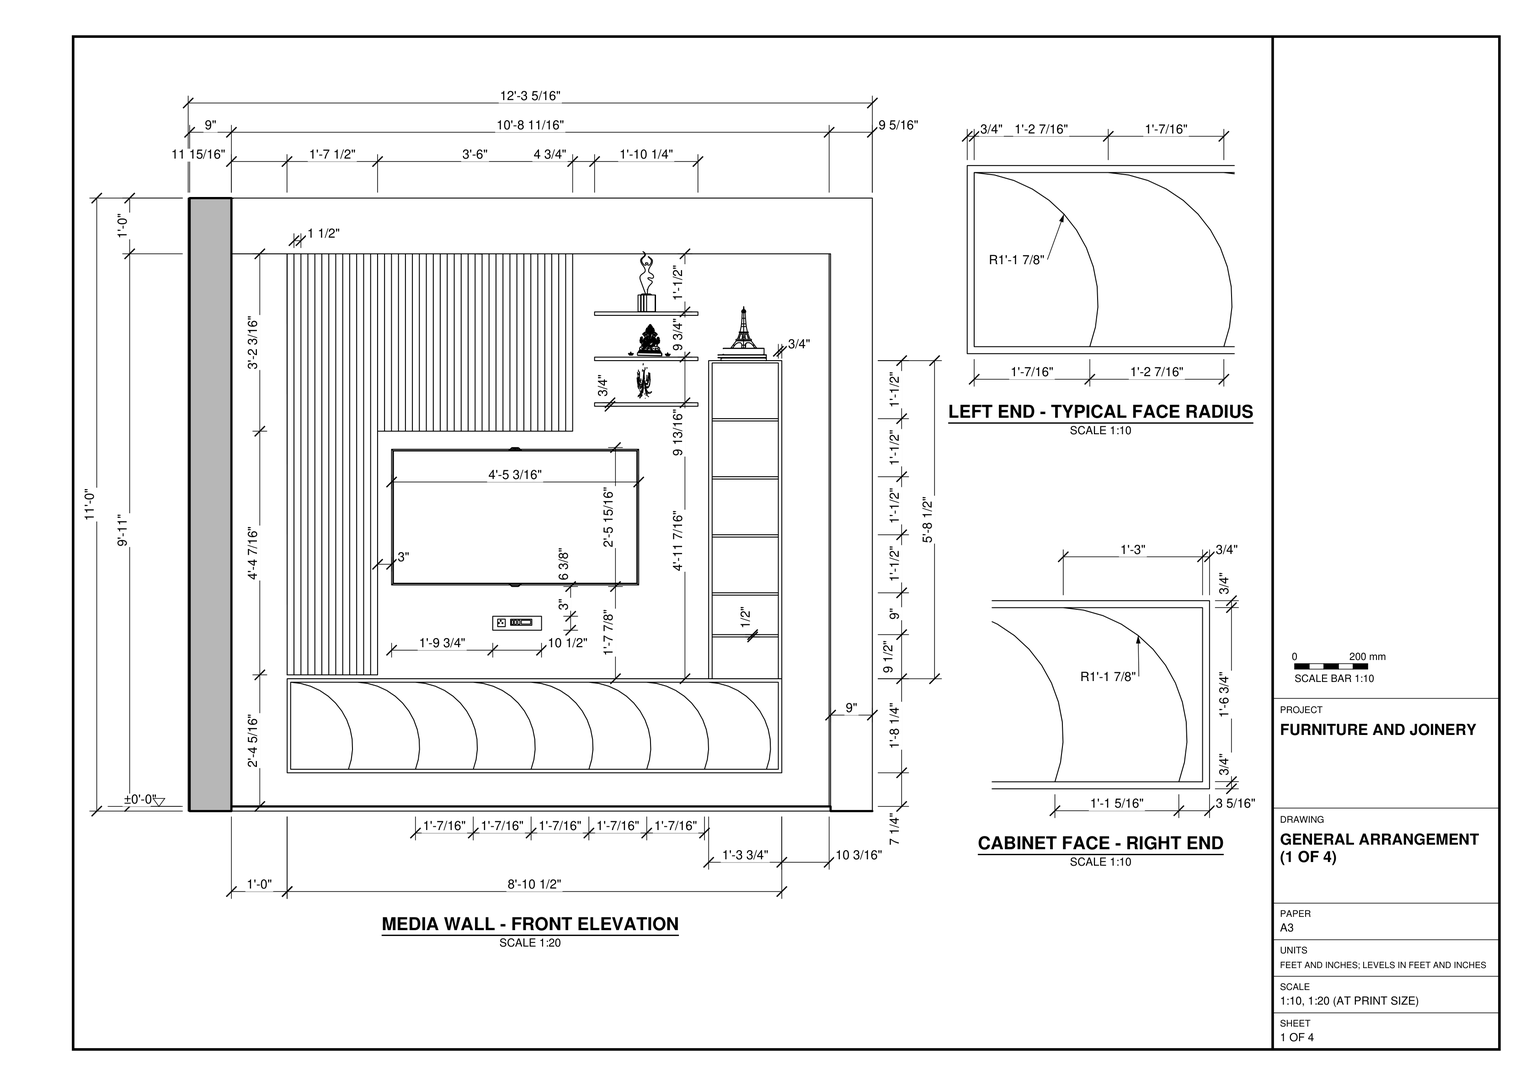
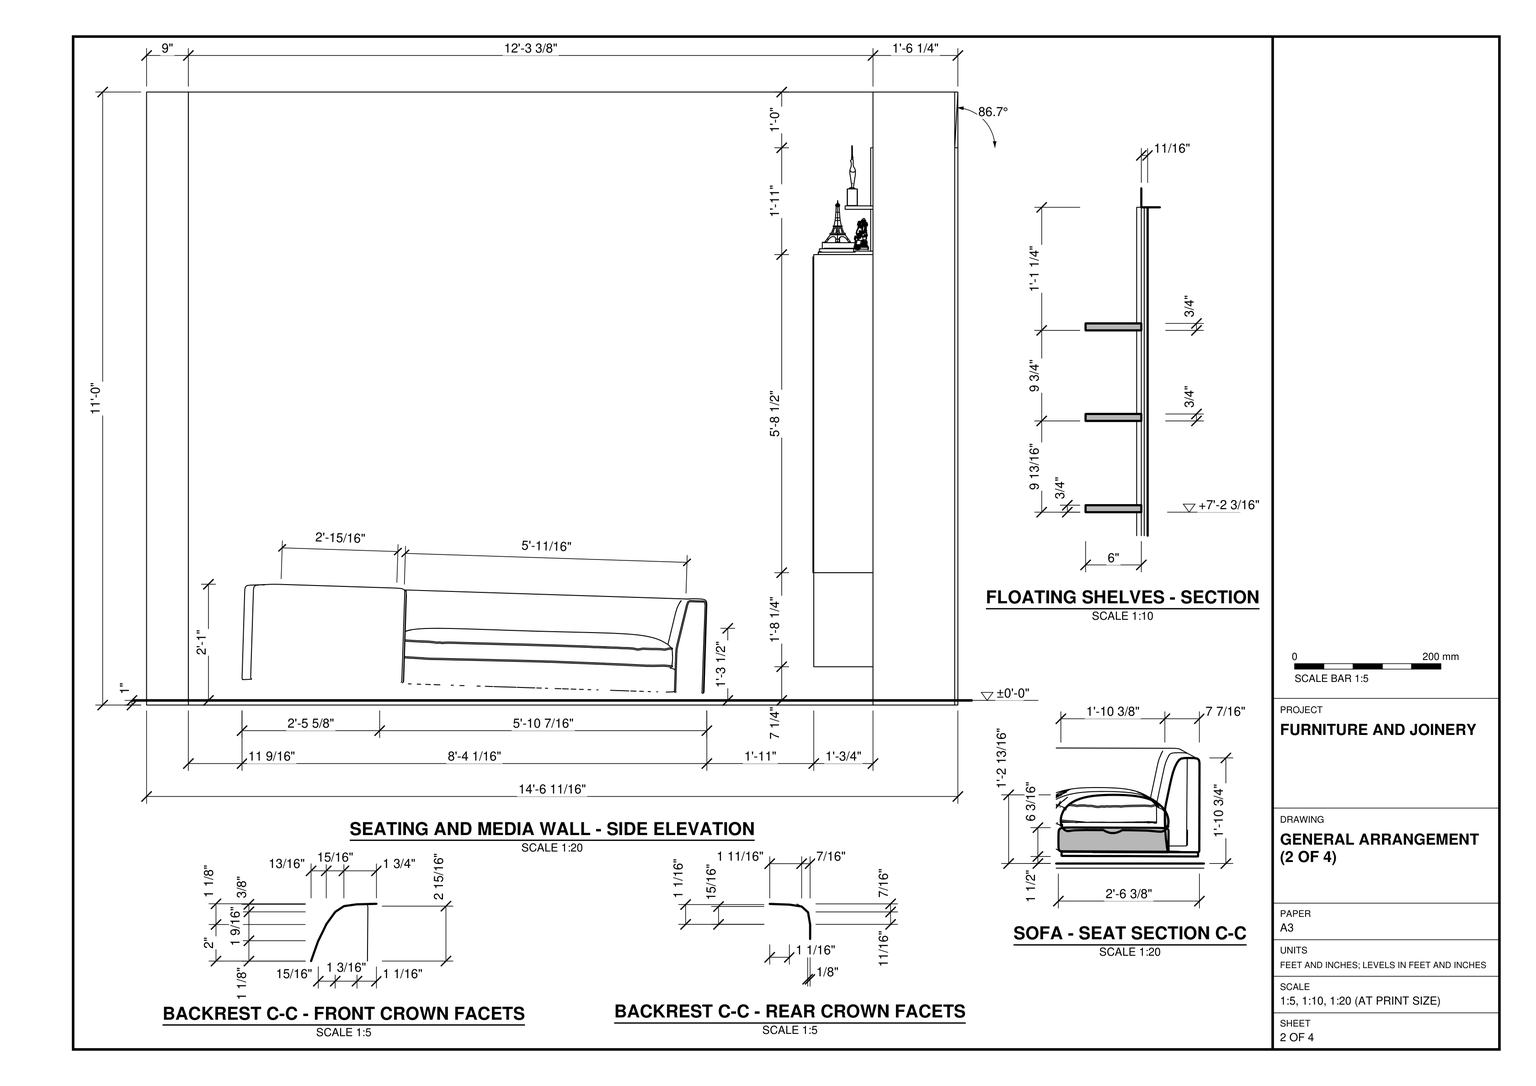
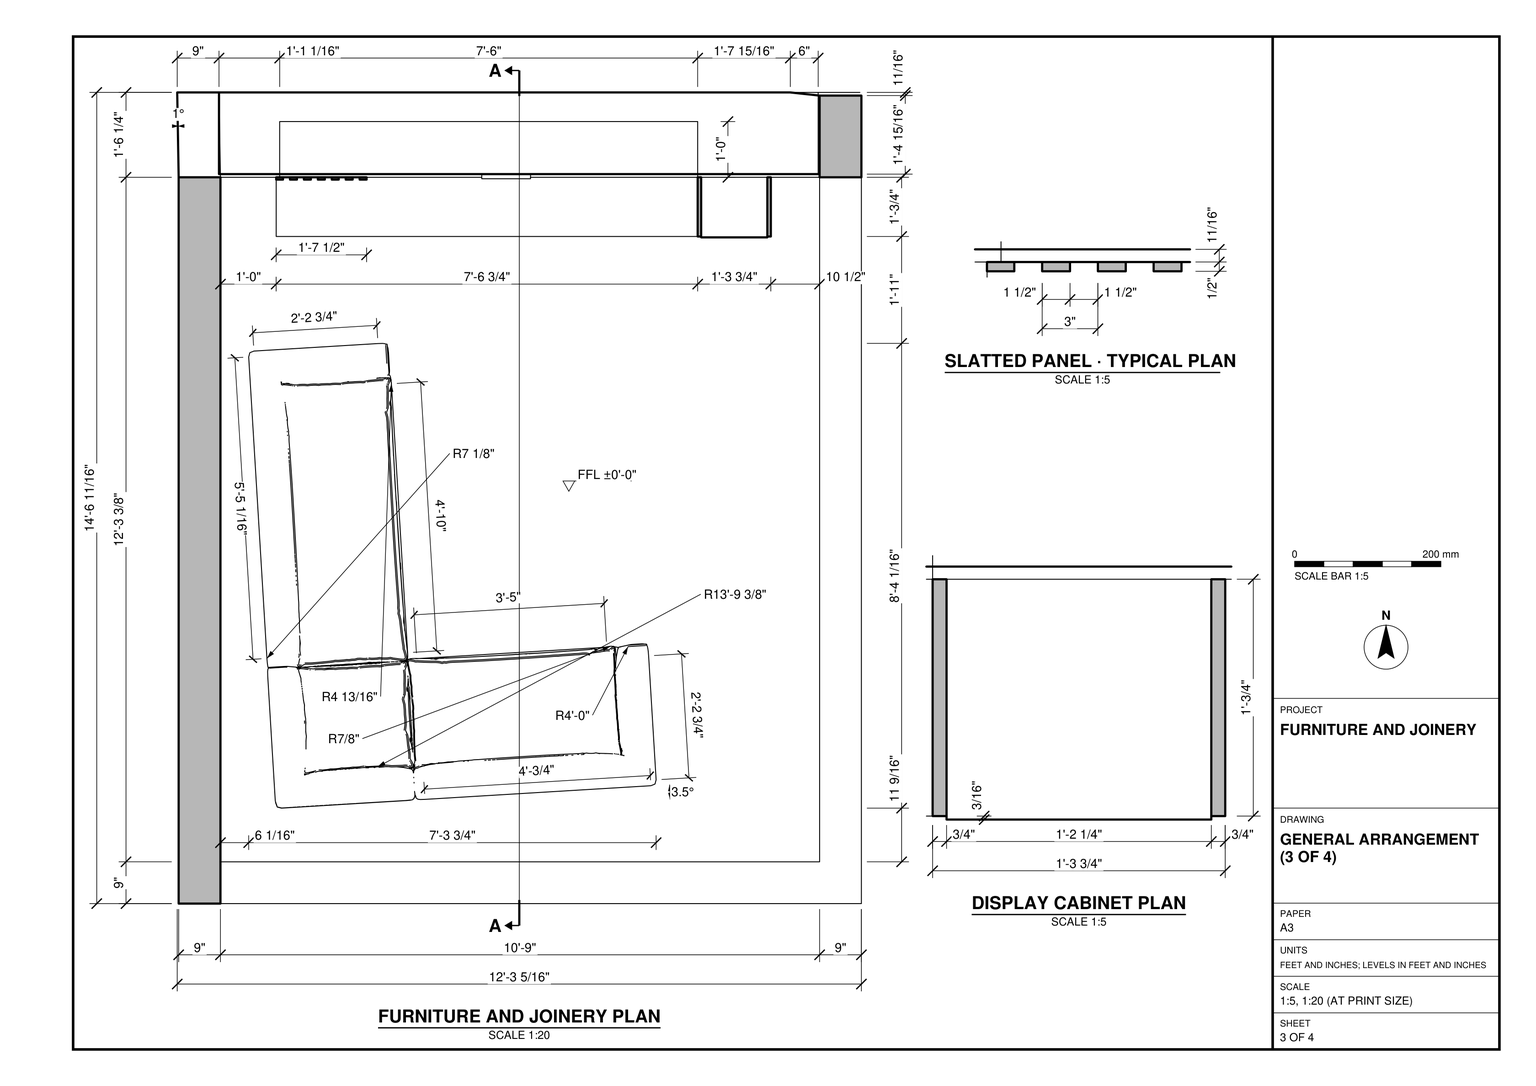
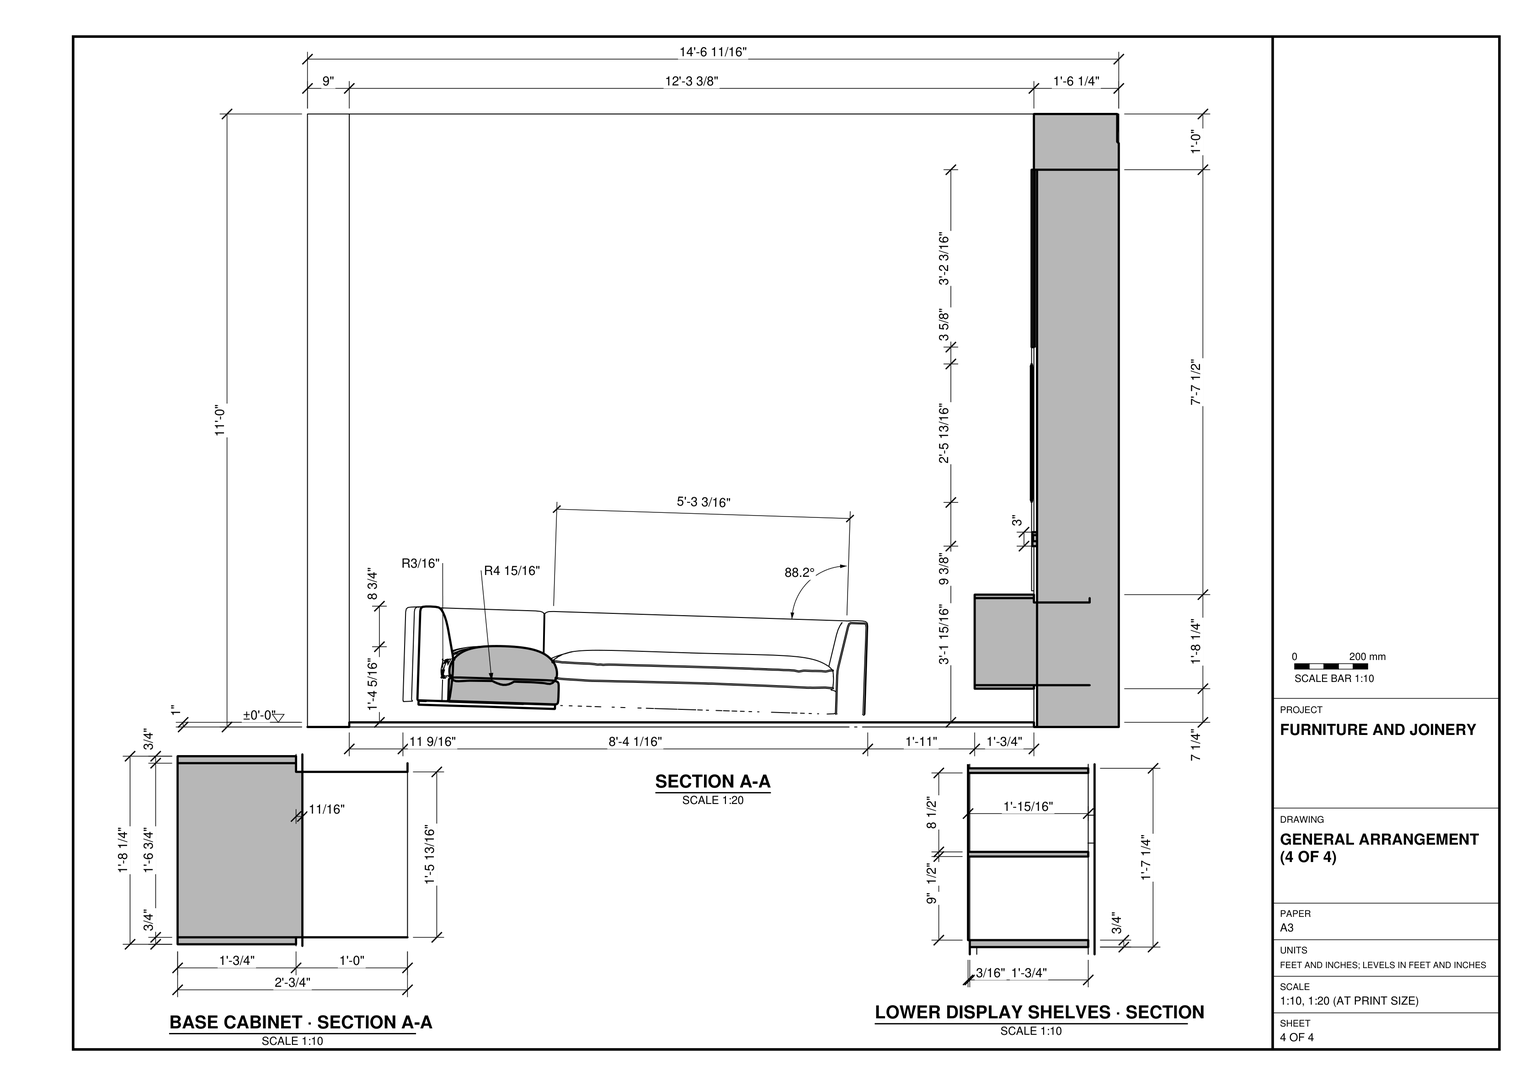
Build the seating area in SketchUp using task_files/diagram_01.pdf. Work in feet and inches. The overall model is 12'-3 5/16" wide by 14'-6 11/16" deep by 11'-2" high, with the finished floor at ±0'-0". Model the floor, the 9" left wall and the media-wall surround, following the plan and sections for their thicknesses and returns.

Set the long base cabinet above the floor and form its fronts with the repeated curved edges shown in the end details. Above it, run the vertical slats down the left side of the screen and across the area above it, keeping the stepped lower edge shown in elevation. Place the outlet plate below the screen. Fit the open display cabinet at the right end of the base cabinet and the three floating shelves between the slatted panel and the display cabinet.

Build the L-shaped sectional sofa with the seat and back profiles shown in section. Position its long leg near the left wall and its shorter leg across the room, preserving the slight angle shown in plan. Decor and loose items may be any suitable library components. Keep shell elements and individual furniture and joinery pieces in separate groups or components, and use components for repeated parts. Save one SketchUp model as output_files/seating_area_with_a_fitted_media_wall.skp.

# SketchUp Ruby script. Lengths in inches.
U = 1.inch
M = Sketchup.active_model
def pt(a) = Geom::Point3d.new(a.map { |v| v * U })
def face(e, loops, mat)
  f = e.add_face(loops[0].map { |a| pt(a) })
  loops[1..].each { |l| e.add_face(l.map { |a| pt(a) }).erase! }
  f.material = f.back_material = mat if mat
  f
end
# faces: each face lists its corners as indices into pts; further lists are holes
def faces(e, pts, list, mat = nil) = list.each { |f| face(e, (f[0].is_a?(Array) ? f : [f]).map { |l| l.map { |i| pts[i] } }, mat) }
# xy, xz, yz: faces in a plane at the given z, y or x. An outline is a flat list of corners, or four numbers for a rectangle; further outlines are holes
def ring(l) = l.size == 4 ? [[l[0], l[1]], [l[2], l[1]], [l[2], l[3]], [l[0], l[3]]] : l.each_slice(2).to_a
def flat(e, list, mat, &to3) = list.each { |f| face(e, (f[0].is_a?(Array) ? f : [f]).map { |l| ring(l).map { |u, v| to3.(u, v) } }, mat) }
def xy(e, z, list, mat = nil) = flat(e, list, mat) { |x, y| [x, y, z] }
def xz(e, y, list, mat = nil) = flat(e, list, mat) { |x, z| [x, y, z] }
def yz(e, x, list, mat = nil) = flat(e, list, mat) { |y, z| [x, y, z] }
def lines(e, pts, list) = list.each { |a, b| e.add_line(pt(pts[a]), pt(pts[b])) }
# prism: a flat outline (further loops are holes) pulled along v
def prism(e, loops, v, mat = nil)
  f = face(e, loops, mat); d = Geom::Vector3d.new(v.map { |x| x * U })
  f.pushpull(f.normal.samedirection?(d) ? d.length : -d.length)
end
def box(e, o, s, mat = nil) = prism(e, [[o, [o[0] + s[0], o[1], o[2]], [o[0] + s[0], o[1] + s[1], o[2]], [o[0], o[1] + s[1], o[2]]]], [0, 0, s[2]], mat)
def at(x, y, z, deg = 0) = Geom::Transformation.translation(pt([x, y, z])) * Geom::Transformation.rotation(ORIGIN, Z_AXIS, deg.degrees)
def axes(o, x, y, z) = Geom::Transformation.new([*x, 0, *y, 0, *z, 0, *pt(o).to_a, 1])
def part(name) = M.definitions.add(name)
# library, detail: a bought-in or finely detailed component or shape, given as its bounding box
def library(name, o, s) = part(name).tap { |d| box(d.entities, o, s) }
def detail(e, o, s) = box(e.add_group.entities, o, s)
def put(e, d, t, mat = nil) = e.add_instance(d, t).tap { |i| i.material = mat if mat }
def group(e, t, mat = nil) = e.add_group.tap { |g| g.transformation = t; g.material = mat if mat }.entities
root = M.entities
M.materials.add("01 - Default2").color = [86, 82, 73]
M.materials.add("6159 FRENCH NUT TREE").color = [139, 95, 49]
M.materials.add("6165 white ash").color = [208, 202, 179]
M.materials.add("6168 WARM ASH").color = [112, 88, 70]
M.materials.add("6184 Aged Elm").color = [88, 77, 65]
M.materials.add("6208 Grey Limed Oak1").color = [150, 141, 131]
M.materials.add("6220 Light Classic Oak").color = [174, 147, 110]
M.materials.add("Heather_Brim1").color = [51, 32, 20]
M.materials.add("Heather_Jeans").color = [86, 117, 147]
M.materials.add("Heather_PantShadow").color = [42, 79, 119]
M.materials.add("Heather_Skin").color = [221, 149, 116]
M.materials.add("Lily_Blonde").color = [204, 166, 108]
M.materials["Lily_Blonde"].alpha = 0.96
M.materials.add("Lily_Light").color = [226, 229, 211]
M.materials.add("Material \#21474428082").color = [180, 179, 173]
M.materials.add("Material \#3a2").color = [91, 47, 14]
M.materials.add("Material~1").color = [48, 234, 223]
M.materials["Material~1"].alpha = 0.35
M.materials.add("[Water Sparkling]").color = [216, 155, 0]
M.materials["[Water Sparkling]"].alpha = 0.6
c1 = library("Flat screen television",[-0.12,1.28,1.14],[53.2,0.41,29.93])
c2 = library("Books with figurine",[-0.1,-1.02,0],[11.3,11.3,11.77])
c3 = library("05 deco",[0,0,0],[11.39,11.6,68.34])
c4 = library("Statue with lamps",[-8.78,0,0],[8.78,25.04,18.65])
c5 = library("Assembly~89_Defintion\#1",[-458.17,-402.78,-169.48],[856.22,828.13,1000])
c6 = library("sofa+(2)",[-221.02,245.34,-31.11],[88.4,103.18,30.14])
xy(root,0,[[0.313,0,9.313,156.404],[0.313,156.404,9.313,156.404,9,174.681,0,174.681],[9.313,156.404,9,174.681,132,174.681,138.313,174,138.313,156.404],[138.313,156.404,147.313,174]],"Lily_Light")
xy(root,0,[[9.313,0,147.313,0,147.313,156.404,138.313,156.404,138.313,9,9.313,9]],"Material \#21474428082")
xy(root,1,[[9.313,9,138.313,156.404]],"Material \#21474428082")
xy(root,8.25,[[21.313,143.654,112.813,156.404],[112.813,143.654,127.813,156.404]])
xy(root,9,[[22.063,143.654,112.063,143.654,112.063,156.404,21.313,156.404,21.313,144.404,22.063,144.404],[112.813,143.654,127.063,156.404],[22.063,156.404,112.063,168.404]])
xy(root,26.8125,[[22.063,156.404,112.063,168.404]])
xy(root,27.75,[[22.063,143.654,22.063,144.404,21.313,144.404,21.313,156.404,112.063,156.404,112.063,143.654],[112.813,143.654,127.063,156.404]])
xy(root,28.5,[[112.813,143.467,127.063,143.654],[112.063,143.654,112.813,156.404],[112.813,143.654,127.063,156.404],[127.063,143.654,127.813,156.404]])
xy(root,28.5,[[21.313,143.654,112.063,156.404]],"6165 white ash")
xy(root,29.338,[[21.313,155.904,22.778,156.404],[24.278,155.904,25.778,156.404],[27.278,155.904,28.778,156.404]],"Heather_Brim1")
xy(root,29.338,[[30.278,155.904,31.778,156.404],[33.278,155.904,34.778,156.404],[36.278,155.904,37.778,156.404],[39.278,155.904,40.778,156.404]],"Lily_Light")
xy(root,37.5,[[112.813,143.467,127.063,156.404]])
xy(root,38,[[112.813,143.467,127.063,156.404]])
xy(root,38.949,[[65.577,156.086,76.077,157.086]])
xy(root,39.71,[[66.641,156.086,68.266,156.273],[66.641,156.273,68.266,157.086]])
xy(root,40.003,[[69.426,156.086,73.989,156.211],[69.426,156.211,73.989,157.086]])
xy(root,41.315,[[69.426,156.086,73.989,156.211],[69.426,156.211,73.989,157.086]])
xy(root,41.335,[[66.641,156.086,68.266,156.273],[66.641,156.273,68.266,157.086]])
xy(root,41.949,[[65.577,156.086,76.077,157.086]])
xy(root,46.5,[[112.813,143.467,127.063,156.404]])
xy(root,47,[[112.813,143.467,127.063,156.404]])
xy(root,59,[[112.813,143.467,127.063,156.404]])
xy(root,59.5,[[112.813,143.467,127.063,156.404]])
xy(root,71.5,[[112.813,143.467,127.063,156.404]])
xy(root,72,[[112.813,143.467,127.063,156.404]])
xy(root,81.804,[[42.278,155.904,43.778,156.404],[45.278,155.904,46.778,156.404],[48.278,155.904,49.778,156.404],[51.278,155.904,52.778,156.404],[54.278,155.904,55.778,156.404],
  [57.278,155.904,58.778,156.404],[60.278,155.904,61.778,156.717],[63.278,155.904,64.778,156.404],[66.278,155.904,67.778,156.404],[69.278,155.904,70.778,156.404],
  [72.278,155.904,73.778,156.404],[75.278,155.904,76.778,156.404],[78.278,155.904,79.778,156.404],[81.278,155.904,82.778,156.404]],"Lily_Light")
xy(root,84,[[112.813,143.467,127.063,156.404]])
xy(root,84.5,[[112.813,143.467,127.063,156.404]])
xy(root,87.175,[[87.5,150.404,109.757,156.404]],"Heather_PantShadow")
xy(root,87.925,[[87.5,150.404,109.757,156.404]],"6208 Grey Limed Oak1")
xy(root,96.5,[[112.813,143.467,127.063,143.654],[112.813,143.654,127.063,156.404]])
xy(root,97,[[112.063,143.654,127.813,156.404]],"6165 white ash")
xy(root,97,[[87.5,150.404,109.757,156.404]],"Heather_PantShadow")
xy(root,97.75,[[87.5,150.404,109.757,156.404]],"6208 Grey Limed Oak1")
xy(root,106.75,[[87.5,150.404,109.757,156.404]],"Heather_PantShadow")
xy(root,107.5,[[87.5,150.404,109.757,156.404]],"6208 Grey Limed Oak1")
xy(root,120,[[21.278,155.904,22.778,156.404],[24.278,155.904,25.778,156.404],[27.278,155.904,28.778,156.404]],"Heather_Brim1")
xy(root,120,[[30.278,155.904,31.778,156.404],[33.278,155.904,34.778,156.404],[36.278,155.904,37.778,156.404],[39.278,155.904,40.778,156.404],[42.278,155.904,43.778,156.404],
  [45.278,155.904,46.778,156.404],[48.278,155.904,49.778,156.404],[51.278,155.904,52.778,156.404],[54.278,155.904,55.778,156.404],[57.278,155.904,58.778,156.404],
  [60.278,155.904,61.778,156.404],[63.278,155.904,64.778,156.404],[66.278,155.904,67.778,156.404],[69.278,155.904,70.778,156.404],[72.278,155.904,73.778,156.404],
  [75.278,155.904,76.778,156.404],[78.278,155.904,79.778,156.404],[81.278,155.904,82.778,156.404],[9.313,156.404,60.278,156.404,60.278,156.717,61.778,156.717,61.778,156.404,138.313,156.404,138.313,174,132,174.681,9,174.681],[60.278,156.404,61.778,156.717]],"Lily_Light")
xy(root,132,[[0.313,0,9.313,156.404],[0.313,156.404,9.313,156.404,9,174.681,0,174.681],[9.313,156.404,147.313,156.404,147.313,174,138.313,174,9,174.681]],"Lily_Light")
xz(root,0,[[0.313,0,9.313,132]],"Lily_Light")
xz(root,9,[[9.313,0,138.313,1]],"Lily_Light")
xz(root,143.467,[[112.813,37.5,127.063,38],[112.813,46.5,127.063,47],[112.813,59,127.063,59.5],[112.813,71.5,127.063,72],[112.813,84,127.063,84.5]],"Lily_Blonde")
xz(root,143.467,[[112.813,28.5,127.063,37.5],[112.813,38,127.063,46.5],[112.813,47,127.063,59],[112.813,59.5,127.063,71.5],[112.813,72,127.063,84],
  [112.813,84.5,127.063,96.5]],"Material~1")
xz(root,143.654,[[124.509,9,127.063,9,127.063,27.75,112.063,27.75,114.232,27.491,116.334,26.896,118.316,25.978,120.129,24.761,121.73,23.274,123.077,21.555,124.138,19.646,124.887,17.594,125.304,15.45,125.38,13.267,125.113,11.099]],"01 - Default2")
xz(root,143.654,[[22.063,9,34.509,9,35.113,11.099,35.38,13.267,35.304,15.45,34.887,17.594,34.138,19.646,33.077,21.555,31.73,23.274,30.129,24.761,28.316,25.978,26.334,26.896,24.232,27.491,22.063,27.75],[34.509,9,48.939,9,49.543,11.099,49.81,13.267,49.734,15.45,49.316,17.594,48.568,19.646,47.507,21.555,46.159,23.274,44.559,24.761,42.745,25.978,40.763,26.896,38.662,27.491,36.493,27.75,22.063,27.75,24.232,27.491,26.334,26.896,28.316,25.978,30.129,24.761,31.73,23.274,33.077,21.555,34.138,19.646,34.887,17.594,35.304,15.45,35.38,13.267,35.113,11.099],[48.939,9,61.385,9,61.989,11.099,62.256,13.267,62.18,15.45,61.762,17.594,61.014,19.646,59.953,21.555,58.605,23.274,57.005,24.761,55.191,25.978,53.209,26.896,51.108,27.491,48.939,27.75,36.493,27.75,38.662,27.491,40.763,26.896,42.745,25.978,44.559,24.761,46.159,23.274,47.507,21.555,48.568,19.646,49.316,17.594,49.734,15.45,49.81,13.267,49.543,11.099],[61.385,9,73.831,9,74.435,11.099,74.702,13.267,74.626,15.45,74.208,17.594,73.46,19.646,72.399,21.555,71.051,23.274,69.451,24.761,67.637,25.978,65.655,26.896,63.554,27.491,61.385,27.75,48.939,27.75,51.108,27.491,53.209,26.896,55.191,25.978,57.005,24.761,58.605,23.274,59.953,21.555,61.014,19.646,61.762,17.594,62.18,15.45,62.256,13.267,61.989,11.099],[73.831,9,86.277,9,86.881,11.099,87.148,13.267,87.072,15.45,86.654,17.594,85.906,19.646,84.845,21.555,83.497,23.274,81.897,24.761,80.083,25.978,78.101,26.896,76,27.491,73.831,27.75,61.385,27.75,63.554,27.491,65.655,26.896,67.637,25.978,69.451,24.761,71.051,23.274,72.399,21.555,73.46,19.646,74.208,17.594,74.626,15.45,74.702,13.267,74.435,11.099],
  [86.277,9,98.723,9,99.327,11.099,99.594,13.267,99.518,15.45,99.1,17.594,98.352,19.646,97.291,21.555,95.943,23.274,94.343,24.761,92.529,25.978,90.547,26.896,88.446,27.491,86.277,27.75,73.831,27.75,76,27.491,78.101,26.896,80.083,25.978,81.897,24.761,83.497,23.274,84.845,21.555,85.906,19.646,86.654,17.594,87.072,15.45,87.148,13.267,86.881,11.099],[98.723,9,111.169,9,111.773,11.099,112.04,13.267,111.964,15.45,111.546,17.594,110.798,19.646,109.737,21.555,108.389,23.274,106.789,24.761,104.975,25.978,102.993,26.896,100.892,27.491,98.723,27.75,86.277,27.75,88.446,27.491,90.547,26.896,92.529,25.978,94.343,24.761,95.943,23.274,97.291,21.555,98.352,19.646,99.1,17.594,99.518,15.45,99.594,13.267,99.327,11.099],[111.169,9,124.509,9,125.113,11.099,125.38,13.267,125.304,15.45,124.887,17.594,124.138,19.646,123.077,21.555,121.73,23.274,120.129,24.761,118.316,25.978,116.334,26.896,114.232,27.491,112.063,27.75,98.723,27.75,100.892,27.491,102.993,26.896,104.975,25.978,106.789,24.761,108.389,23.274,109.737,21.555,110.798,19.646,111.546,17.594,111.964,15.45,112.04,13.267,111.773,11.099]],"6220 Light Classic Oak")
xz(root,143.654,[[[21.313,8.25,127.813,28.5],[22.063,9,127.063,27.75]],[112.063,28.5,112.813,28.5,112.813,96.5,127.063,96.5,127.063,28.5,127.813,28.5,127.813,97,112.063,97]],"Lily_Blonde")
xz(root,144.404,[[21.313,9,22.063,27.75]])
xz(root,150.404,[[87.5,87.175,109.757,87.925],[87.5,97,109.757,97.75],[87.5,106.75,109.757,107.5]],"Lily_Blonde")
xz(root,155.904,[[21.313,29.338,22.778,120],[24.278,29.338,25.778,120],[27.278,29.338,28.778,120],[30.278,29.338,31.778,120],[33.278,29.338,34.778,120],
  [36.278,29.338,37.778,120],[39.278,29.338,40.778,120],[42.278,81.804,43.778,120],[45.278,81.804,46.778,120],[48.278,81.804,49.778,120],
  [51.278,81.804,52.778,120],[54.278,81.804,55.778,120],[57.278,81.804,58.778,120],[60.278,81.804,61.778,120],[63.278,81.804,64.778,120],
  [66.278,81.804,67.778,120],[69.278,81.804,70.778,120],[72.278,81.804,73.778,120],[75.278,81.804,76.778,120],[78.278,81.804,79.778,120],
  [81.278,81.804,82.778,120]],"6165 white ash")
xz(root,155.904,[[21.313,29.338,21.313,120,21.278,120]],"Heather_Brim1")
xz(root,155.904,[[84.278,120.003,85.725,120.005]],"Lily_Light")
xz(root,156.086,[[[65.577,38.949,76.077,41.949],[69.426,40.003,73.989,41.315],[66.641,39.71,68.266,41.335]]])
xz(root,156.211,[[[69.426,40.003,73.989,41.315],[71.728,40.271,73.728,41.084],[70.249,40.228,70.687,41.103],[70.973,40.219,71.411,41.094],[69.637,40.212,70.012,41.087]],[69.637,40.212,70.012,41.087],[70.973,40.219,71.411,41.094],[70.249,40.228,70.687,41.103],[71.728,40.271,73.728,41.084]])
xz(root,156.273,[[[66.641,39.71,68.266,41.335],[66.894,40.368,66.861,40.371,66.83,40.381,66.803,40.4,66.782,40.424,66.768,40.454,66.761,40.486,66.764,40.518,66.774,40.549,66.793,40.576,66.817,40.598,66.847,40.612,66.879,40.618,66.911,40.616,66.942,40.605,66.969,40.587,66.99,40.562,67.005,40.533,67.011,40.501,67.009,40.468,66.998,40.4375,66.98,40.41,66.955,40.389,66.926,40.375],[67.288,40.849,67.255,40.854,67.225,40.866,67.199,40.886,67.179,40.912,67.167,40.942,67.163,40.974,67.167,41.007,67.179,41.037,67.199,41.063,67.225,41.083,67.255,41.095,67.288,41.099,67.32,41.095,67.35,41.083,67.376,41.063,67.396,41.037,67.408,41.007,67.413,40.974,67.408,40.942,67.396,40.912,67.376,40.886,67.35,40.866,67.32,40.854],[67.671,40.373,67.64,40.377,67.611,40.389,67.586,40.408,67.567,40.433,67.555,40.462,67.551,40.493,67.555,40.524,67.567,40.553,67.586,40.578,67.611,40.598,67.64,40.61,67.671,40.614,67.702,40.61,67.731,40.598,67.756,40.578,67.775,40.553,67.787,40.524,67.791,40.493,67.787,40.462,67.775,40.433,67.756,40.408,67.731,40.389,67.702,40.377]]])
xz(root,156.398,[[66.894,40.368,66.926,40.375,66.955,40.389,66.98,40.41,66.998,40.4375,67.009,40.468,67.011,40.501,67.005,40.533,66.99,40.562,66.969,40.587,66.942,40.605,66.911,40.616,66.879,40.618,66.847,40.612,66.817,40.598,66.793,40.576,66.774,40.549,66.764,40.518,66.761,40.486,66.768,40.454,66.782,40.424,66.803,40.4,66.83,40.381,66.861,40.371],[67.671,40.373,67.702,40.377,67.731,40.389,67.756,40.408,67.775,40.433,67.787,40.462,67.791,40.493,67.787,40.524,67.775,40.553,67.756,40.578,67.731,40.598,67.702,40.61,67.671,40.614,67.64,40.61,67.611,40.598,67.586,40.578,67.567,40.553,67.555,40.524,67.551,40.493,67.555,40.462,67.567,40.433,67.586,40.408,67.611,40.389,67.64,40.377]])
xz(root,156.404,[[21.313,8.25,21.313,9,112.063,9,112.063,27.75,21.313,27.75,21.313,28.5,112.813,28.5,112.813,8.25],[112.813,8.25,112.813,9,127.063,9,127.063,28.5,127.813,28.5,127.813,8.25],[21.313,9,22.063,26.8125],[21.313,26.8125,112.063,27.75],[112.813,27.75,127.063,28.5],
  [112.063,28.5,112.063,97,127.813,97,127.813,28.5,127.063,28.5,127.063,96.5,112.813,96.5,112.813,28.5],[112.813,37.5,127.063,38],[112.813,46.5,127.063,47],[112.813,59,127.063,59.5],[112.813,71.5,127.063,72],
  [112.813,84,127.063,84.5]])
xz(root,156.404,[[0.313,0,0.313,132,147.313,132,147.313,0,138.313,0,138.313,120,9.313,120,9.313,0]],"6168 WARM ASH")
xz(root,156.404,[[25.778,29.338,27.278,120],[28.778,29.338,30.278,120],[31.778,29.338,33.278,120],[34.778,29.338,36.278,120],[37.778,29.338,39.278,120],
  [40.778,81.804,42.278,120],[43.778,81.804,45.278,120],[46.778,81.804,48.278,120],[49.778,81.804,51.278,120],[52.778,81.804,54.278,120],
  [55.778,81.804,57.278,120],[58.778,81.804,60.278,120],[64.778,81.804,66.278,120],[67.778,81.804,69.278,120],[70.778,81.804,72.278,120],
  [73.778,81.804,75.278,120],[76.778,81.804,78.278,120],[79.778,81.804,81.278,120]],"6184 Aged Elm")
xz(root,156.404,[[27.278,29.338,28.778,120]],"Heather_Brim1")
xz(root,156.404,[[87.5,87.175,109.757,87.925],[87.5,97,109.757,97.75],[87.5,106.75,109.757,107.5]],"Heather_PantShadow")
xz(root,156.404,[[9.313,0,138.313,1],[21.313,29.338,21.278,120,22.778,120,22.778,29.338],[24.278,29.338,25.778,120],[30.278,29.338,31.778,120],[33.278,29.338,34.778,120],
  [36.278,29.338,37.778,120],[39.278,29.338,40.778,120],[42.278,81.804,43.778,120],[45.278,81.804,46.778,120],[48.278,81.804,49.778,120],
  [51.278,81.804,52.778,120],[54.278,81.804,55.778,120],[57.278,81.804,58.778,120],[63.278,81.804,64.778,120],[66.278,81.804,67.778,120],
  [69.278,81.804,70.778,120],[72.278,81.804,73.778,120],[75.278,81.804,76.778,120],[78.278,81.804,79.778,120],[81.278,81.804,82.778,120]],"Lily_Light")
xz(root,156.404,[[22.778,29.338,24.278,120]],"[Water Sparkling]")
xz(root,156.648,[[67.288,40.849,67.32,40.854,67.35,40.866,67.376,40.886,67.396,40.912,67.408,40.942,67.413,40.974,67.408,41.007,67.396,41.037,67.376,41.063,67.35,41.083,67.32,41.095,67.288,41.099,67.255,41.095,67.225,41.083,67.199,41.063,67.179,41.037,67.167,41.007,67.163,40.974,67.167,40.942,67.179,40.912,67.199,40.886,67.225,40.866,67.255,40.854]])
xz(root,156.717,[[60.278,81.804,61.778,120]],"Lily_Light")
xz(root,157.086,[[[65.577,38.949,76.077,41.949],[69.426,40.003,73.989,41.315],[66.641,39.71,68.266,41.335]]])
xz(root,168.404,[[22.063,26.8125,112.063,27.75]])
xz(root,174,[[138.313,0,147.313,132]],"Lily_Light")
xz(root,174.681,[[0,0,0,132,9,132,9,120,132,120,132,0],[9,120,9,132,132,120]],"Lily_Light")
yz(root,0.313,[[0,0,156.404,132]],"Lily_Light")
yz(root,9.313,[[0,0,9,132],[9,0,156.404,1]],"Lily_Light")
yz(root,9.313,[[9,1,156.404,132]],"Material \#3a2")
yz(root,21.313,[[143.654,8.25,156.404,9]])
yz(root,21.313,[[144.404,9,156.404,27.75],[143.654,27.75,156.404,28.5]],"6208 Grey Limed Oak1")
yz(root,21.313,[[143.654,9,144.404,27.75]],"Heather_Skin")
yz(root,22.063,[[143.654,9,144.404,27.75],[156.404,9,168.404,26.8125]])
yz(root,22.778,[[155.904,29.338,156.404,120]],"6159 FRENCH NUT TREE")
yz(root,24.278,[[155.904,29.338,156.404,120]],"6159 FRENCH NUT TREE")
yz(root,25.778,[[155.904,29.338,156.404,120]],"6159 FRENCH NUT TREE")
yz(root,27.278,[[155.904,29.338,156.404,120]],"6159 FRENCH NUT TREE")
yz(root,28.778,[[155.904,29.338,156.404,120]],"6159 FRENCH NUT TREE")
yz(root,30.278,[[155.904,29.338,156.404,120]],"6159 FRENCH NUT TREE")
yz(root,31.778,[[155.904,29.338,156.404,120]],"6159 FRENCH NUT TREE")
yz(root,33.278,[[155.904,29.338,156.404,120]],"6159 FRENCH NUT TREE")
yz(root,34.778,[[155.904,29.338,156.404,120]],"6159 FRENCH NUT TREE")
yz(root,36.278,[[155.904,29.338,156.404,120]],"6159 FRENCH NUT TREE")
yz(root,37.778,[[155.904,29.338,156.404,120]],"6159 FRENCH NUT TREE")
yz(root,39.278,[[155.904,29.338,156.404,120]],"6159 FRENCH NUT TREE")
yz(root,40.778,[[155.904,29.338,156.404,120]],"6159 FRENCH NUT TREE")
yz(root,42.278,[[155.904,81.804,156.404,120]],"6159 FRENCH NUT TREE")
yz(root,43.778,[[155.904,81.804,156.404,120]],"6159 FRENCH NUT TREE")
yz(root,45.278,[[155.904,81.804,156.404,120]],"6159 FRENCH NUT TREE")
yz(root,46.778,[[155.904,81.804,156.404,120]],"6159 FRENCH NUT TREE")
yz(root,48.278,[[155.904,81.804,156.404,120]],"6159 FRENCH NUT TREE")
yz(root,49.778,[[155.904,81.804,156.404,120]],"6159 FRENCH NUT TREE")
yz(root,51.278,[[155.904,81.804,156.404,120]],"6159 FRENCH NUT TREE")
yz(root,52.778,[[155.904,81.804,156.404,120]],"6159 FRENCH NUT TREE")
yz(root,54.278,[[155.904,81.804,156.404,120]],"6159 FRENCH NUT TREE")
yz(root,55.778,[[155.904,81.804,156.404,120]],"6159 FRENCH NUT TREE")
yz(root,57.278,[[155.904,81.804,156.404,120]],"6159 FRENCH NUT TREE")
yz(root,58.778,[[155.904,81.804,156.404,120]],"6159 FRENCH NUT TREE")
yz(root,60.278,[[155.904,81.804,156.404,120],[156.404,81.804,156.717,120]],"6159 FRENCH NUT TREE")
yz(root,61.778,[[155.904,81.804,156.717,120]],"6159 FRENCH NUT TREE")
yz(root,63.278,[[155.904,81.804,156.404,120]],"6159 FRENCH NUT TREE")
yz(root,64.778,[[155.904,81.804,156.404,120]],"6159 FRENCH NUT TREE")
yz(root,65.577,[[156.086,38.949,157.086,41.949]])
yz(root,66.278,[[155.904,81.804,156.404,120]],"6159 FRENCH NUT TREE")
yz(root,66.641,[[156.086,39.71,156.273,41.335],[156.273,39.71,157.086,41.335]])
yz(root,67.778,[[155.904,81.804,156.404,120]],"6159 FRENCH NUT TREE")
yz(root,68.266,[[156.086,39.71,156.273,41.335],[156.273,39.71,157.086,41.335]])
yz(root,69.278,[[155.904,81.804,156.404,120]],"6159 FRENCH NUT TREE")
yz(root,69.426,[[156.086,40.003,156.211,41.315],[156.211,40.003,157.086,41.315]])
yz(root,70.778,[[155.904,81.804,156.404,120]],"6159 FRENCH NUT TREE")
yz(root,72.278,[[155.904,81.804,156.404,120]],"6159 FRENCH NUT TREE")
yz(root,73.778,[[155.904,81.804,156.404,120]],"6159 FRENCH NUT TREE")
yz(root,73.989,[[156.086,40.003,156.211,41.315],[156.211,40.003,157.086,41.315]])
yz(root,75.278,[[155.904,81.804,156.404,120]],"6159 FRENCH NUT TREE")
yz(root,76.077,[[156.086,38.949,157.086,41.949]])
yz(root,76.778,[[155.904,81.804,156.404,120]],"6159 FRENCH NUT TREE")
yz(root,78.278,[[155.904,81.804,156.404,120]],"6159 FRENCH NUT TREE")
yz(root,79.778,[[155.904,81.804,156.404,120]],"6159 FRENCH NUT TREE")
yz(root,81.278,[[155.904,81.804,156.404,120]],"6159 FRENCH NUT TREE")
yz(root,82.778,[[155.904,81.804,156.404,120]],"6159 FRENCH NUT TREE")
yz(root,87.5,[[150.404,87.175,156.404,87.925],[150.404,97,156.404,97.75],[150.404,106.75,156.404,107.5]],"Heather_PantShadow")
yz(root,109.757,[[150.404,87.175,156.404,87.925],[150.404,97,156.404,97.75],[150.404,106.75,156.404,107.5]],"Heather_PantShadow")
yz(root,112.063,[[156.404,9,168.404,26.8125]])
yz(root,112.063,[[143.654,28.5,156.404,97]],"6208 Grey Limed Oak1")
yz(root,112.813,[[143.467,28.5,143.654,37.5],[143.654,28.5,156.404,37.5],[143.467,37.5,143.654,38],[143.654,37.5,156.404,38],[143.467,38,143.654,46.5],
  [143.654,38,156.404,46.5],[143.467,46.5,143.654,47],[143.654,46.5,156.404,47],[143.467,47,143.654,59],[143.654,47,156.404,59],
  [143.467,59,143.654,59.5],[143.654,59,156.404,59.5],[143.467,59.5,143.654,71.5],[143.654,59.5,156.404,71.5],[143.467,71.5,143.654,72],
  [143.654,71.5,156.404,72],[143.467,72,143.654,84],[143.654,72,156.404,84],[143.467,84,143.654,84.5],[143.654,84,156.404,84.5],
  [143.467,84.5,143.654,96.5],[143.654,84.5,156.404,96.5]])
yz(root,127.063,[[143.654,9,156.404,27.75],[143.467,28.5,143.654,37.5],[143.654,28.5,156.404,37.5],[143.467,37.5,143.654,38],[143.654,37.5,156.404,38],
  [143.467,38,143.654,46.5],[143.654,38,156.404,46.5],[143.467,46.5,143.654,47],[143.654,46.5,156.404,47],[143.467,47,143.654,59],
  [143.654,47,156.404,59],[143.467,59,143.654,59.5],[143.654,59,156.404,59.5],[143.467,59.5,143.654,71.5],[143.654,59.5,156.404,71.5],
  [143.467,71.5,143.654,72],[143.654,71.5,156.404,72],[143.467,72,143.654,84],[143.654,72,156.404,84],[143.467,84,143.654,84.5],
  [143.654,84,156.404,84.5],[143.467,84.5,143.654,96.5],[143.654,84.5,156.404,96.5]])
yz(root,127.813,[[143.654,8.25,156.404,28.5],[143.654,28.5,156.404,97]],"01 - Default2")
yz(root,138.313,[[9,0,156.404,1],[156.404,0,174,120]],"Lily_Light")
yz(root,147.313,[[156.404,0,174,132]],"Lily_Light")
p = [[0.313,156.404,132],[0,174.681,132],[0,174.681,0],[0.313,156.404,0],[132,174.681,0],[132,174.681,120],
  [138.313,174,120],[138.313,174,0],[21.278,156.404,120],[21.313,156.404,29.338],[21.313,155.904,29.338],[21.278,155.904,120],
  [66.768,156.273,40.454],[66.782,156.273,40.424],[66.782,156.398,40.424],[66.768,156.398,40.454],[66.803,156.273,40.4],[66.803,156.398,40.4],
  [66.83,156.273,40.381],[66.83,156.398,40.381],[66.861,156.273,40.371],[66.861,156.398,40.371],[66.894,156.273,40.368],[66.894,156.398,40.368],
  [66.926,156.273,40.375],[66.926,156.398,40.375],[66.955,156.273,40.389],[66.955,156.398,40.389],[66.98,156.273,40.41],[66.98,156.398,40.41],
  [66.998,156.273,40.4375],[66.998,156.398,40.4375],[67.009,156.273,40.468],[67.009,156.398,40.468],[67.555,156.273,40.462],[67.567,156.273,40.433],
  [67.567,156.398,40.433],[67.555,156.398,40.462],[67.586,156.273,40.408],[67.586,156.398,40.408],[67.611,156.273,40.389],[67.611,156.398,40.389],
  [67.64,156.273,40.377],[67.64,156.398,40.377],[67.671,156.273,40.373],[67.671,156.398,40.373],[67.702,156.273,40.377],[67.702,156.398,40.377],
  [67.731,156.273,40.389],[67.731,156.398,40.389],[67.756,156.273,40.408],[67.756,156.398,40.408],[67.775,156.273,40.433],[67.775,156.398,40.433],
  [67.787,156.273,40.462],[67.787,156.398,40.462],[66.793,156.273,40.576],[66.774,156.273,40.549],[66.774,156.398,40.549],[66.793,156.398,40.576],
  [66.764,156.273,40.518],[66.764,156.398,40.518],[66.761,156.273,40.486],[66.761,156.398,40.486],[67.011,156.273,40.501],[67.011,156.398,40.501],
  [67.005,156.273,40.533],[67.005,156.398,40.533],[66.99,156.273,40.562],[66.99,156.398,40.562],[67.567,156.273,40.553],[67.555,156.273,40.524],
  [67.555,156.398,40.524],[67.567,156.398,40.553],[67.551,156.273,40.493],[67.551,156.398,40.493],[67.791,156.273,40.493],[67.791,156.398,40.493],
  [67.787,156.273,40.524],[67.787,156.398,40.524],[67.775,156.273,40.553],[67.775,156.398,40.553],[66.879,156.273,40.618],[66.847,156.273,40.612],
  [66.847,156.398,40.612],[66.879,156.398,40.618],[66.817,156.273,40.598],[66.817,156.398,40.598],[66.969,156.273,40.587],[66.942,156.273,40.605],
  [66.942,156.398,40.605],[66.969,156.398,40.587],[66.911,156.273,40.616],[66.911,156.398,40.616],[67.671,156.273,40.614],[67.64,156.273,40.61],
  [67.64,156.398,40.61],[67.671,156.398,40.614],[67.611,156.273,40.598],[67.611,156.398,40.598],[67.586,156.273,40.578],[67.586,156.398,40.578],
  [67.702,156.273,40.61],[67.702,156.398,40.61],[67.756,156.273,40.578],[67.731,156.273,40.598],[67.731,156.398,40.598],[67.756,156.398,40.578],
  [67.255,156.273,40.854],[67.288,156.273,40.849],[67.288,156.648,40.849],[67.255,156.648,40.854],[67.32,156.273,40.854],[67.32,156.648,40.854],
  [67.163,156.273,40.974],[67.167,156.273,40.942],[67.167,156.648,40.942],[67.163,156.648,40.974],[67.179,156.273,40.912],[67.179,156.648,40.912],
  [67.199,156.273,40.886],[67.199,156.648,40.886],[67.225,156.273,40.866],[67.225,156.648,40.866],[67.35,156.273,40.866],[67.35,156.648,40.866],
  [67.376,156.273,40.886],[67.376,156.648,40.886],[67.396,156.273,40.912],[67.396,156.648,40.912],[67.408,156.273,40.942],[67.408,156.648,40.942],
  [67.413,156.273,40.974],[67.413,156.648,40.974],[67.199,156.273,41.063],[67.179,156.273,41.037],[67.179,156.648,41.037],[67.199,156.648,41.063],
  [67.167,156.273,41.007],[67.167,156.648,41.007],[67.408,156.273,41.007],[67.396,156.273,41.037],[67.396,156.648,41.037],[67.408,156.648,41.007],
  [67.376,156.273,41.063],[67.376,156.648,41.063],[67.255,156.273,41.095],[67.225,156.273,41.083],[67.225,156.648,41.083],[67.255,156.648,41.095],
  [67.35,156.273,41.083],[67.32,156.273,41.095],[67.32,156.648,41.095],[67.35,156.648,41.083],[67.288,156.273,41.099],[67.288,156.648,41.099],
  [61.778,156.717,120],[63.278,156.404,119.952],[63.278,156.404,81.804],[61.778,156.717,81.804],[85.725,156.404,120],[84.278,156.404,120],
  [84.278,155.904,120.005],[85.725,155.904,120.005],[9.313,156.404,120],[9,174.681,120],[9,174.681,132],[9.313,156.404,132],
  [138.313,174,132],[21.278,156.404,29.338],[21.313,155.904,120],[21.313,155.904,120.003]]
faces(root,p,[[0,1,2,3],[4,5,6,7],[160,161,162,163],[6,5,166],[168,6,166]],"Lily_Light")
faces(root,p,[[8,9,10,11]],"6159 FRENCH NUT TREE")
faces(root,p,[[12,13,14,15],[13,16,17,14],[16,18,19,17],[18,20,21,19],[20,22,23,21],[22,24,25,23],[24,26,27,25],[26,28,29,27],
  [28,30,31,29],[30,32,33,31],[34,35,36,37],[35,38,39,36],[38,40,41,39],[40,42,43,41],[42,44,45,43],[44,46,47,45],
  [46,48,49,47],[48,50,51,49],[50,52,53,51],[52,54,55,53],[56,57,58,59],[57,60,61,58],[60,62,63,61],[62,12,15,63],
  [32,64,65,33],[64,66,67,65],[66,68,69,67],[70,71,72,73],[71,74,75,72],[74,34,37,75],[54,76,77,55],[76,78,79,77],
  [78,80,81,79],[82,83,84,85],[83,86,87,84],[86,56,59,87],[88,89,90,91],[89,92,93,90],[92,82,85,93],[68,88,91,69],
  [94,95,96,97],[95,98,99,96],[98,100,101,99],[100,70,73,101],[102,94,97,103],[104,105,106,107],[105,102,103,106],[80,104,107,81],
  [108,109,110,111],[109,112,113,110],[114,115,116,117],[115,118,119,116],[118,120,121,119],[120,122,123,121],[122,108,111,123],[112,124,125,113],
  [124,126,127,125],[126,128,129,127],[128,130,131,129],[130,132,133,131],[134,135,136,137],[135,138,139,136],[138,114,117,139],[140,141,142,143],
  [141,144,145,142],[132,140,143,133],[146,147,148,149],[147,134,137,148],[150,151,152,153],[151,154,155,152],[154,146,149,155],[144,150,153,145]])
faces(root,p,[[156,157,158,159]],"6184 Aged Elm")
faces(root,p,[[164,165,166,167]],"Heather_Jeans")
lines(root,p,[[9,169],[170,171]])
put(root,c1,at(43.92,154.46,47.21))
put(root,c2,at(114.06,144.17,96.88))
put(root,c3,axes([96.86,150.85,107.57],[0.33067,0,0],[0,0.18896,0],[0,0,0.18896]))
put(root,c4,axes([94.75,152.32,98.21],[-0.00883,-0.35984,0.00607],[0.35983,-0.00894,-0.00671],[0.00686,0.0059,0.35989]))
put(root,c5,axes([98.1,154.74,94.97],[-0.00414,0,0],[0,-0.00829,0],[0,0,-0.00829]))
put(root,c6,axes([236.39,-224.03,36.75],[0.99921,0.00395,0.03953],[-0.00373,0.99998,-0.00576],[-0.03955,0.00561,0.9992]),"Material \#3a2")
g1 = group(root,at(9,157.09,0),"6168 WARM ASH")
xz(g1,0,[[0,0,129,120]])
xz(g1,17.6,[[0,0,123,120]])
yz(g1,0,[[0,0,17.6,120]])
p = [[0,17.6,120],[0,17.6,132],[129,17.6,0],[123,17.6,0],[138,17.6,0],[129,0,0]]
lines(g1,p,[[0,1],[2,3],[2,4],[5,2]])
